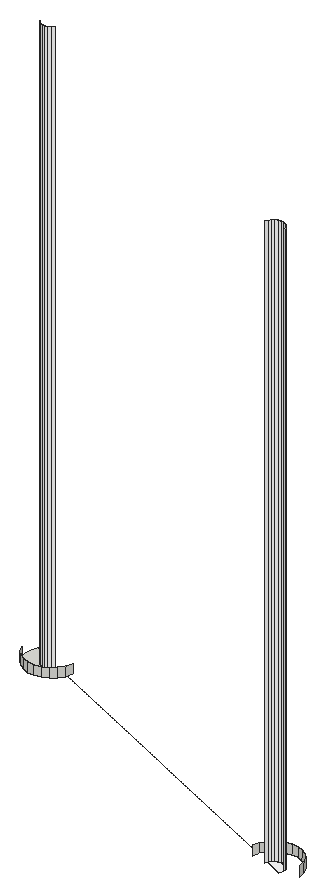
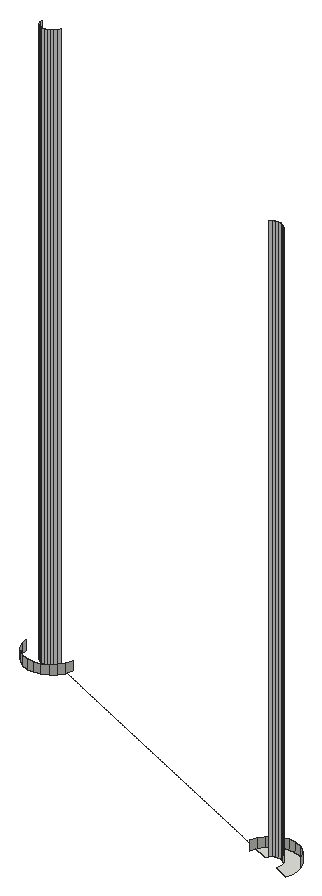
# SketchUp Ruby script. Lengths in inches.
U = 1.inch
M = Sketchup.active_model
def pt(a) = Geom::Point3d.new(a.map { |v| v * U })
def face(e, loops, mat)
  f = e.add_face(loops[0].map { |a| pt(a) })
  loops[1..].each { |l| e.add_face(l.map { |a| pt(a) }).erase! }
  f.material = f.back_material = mat if mat
  f
end
# faces: each face lists its corners as indices into pts; further lists are holes
def faces(e, pts, list, mat = nil) = list.each { |f| face(e, (f[0].is_a?(Array) ? f : [f]).map { |l| l.map { |i| pts[i] } }, mat) }
# xy, xz, yz: faces in a plane at the given z, y or x. An outline is a flat list of corners, or four numbers for a rectangle; further outlines are holes
def ring(l) = l.size == 4 ? [[l[0], l[1]], [l[2], l[1]], [l[2], l[3]], [l[0], l[3]]] : l.each_slice(2).to_a
def flat(e, list, mat, &to3) = list.each { |f| face(e, (f[0].is_a?(Array) ? f : [f]).map { |l| ring(l).map { |u, v| to3.(u, v) } }, mat) }
def xy(e, z, list, mat = nil) = flat(e, list, mat) { |x, y| [x, y, z] }
def xz(e, y, list, mat = nil) = flat(e, list, mat) { |x, z| [x, y, z] }
def yz(e, x, list, mat = nil) = flat(e, list, mat) { |y, z| [x, y, z] }
def lines(e, pts, list) = list.each { |a, b| e.add_line(pt(pts[a]), pt(pts[b])) }
# prism: a flat outline (further loops are holes) pulled along v
def prism(e, loops, v, mat = nil)
  f = face(e, loops, mat); d = Geom::Vector3d.new(v.map { |x| x * U })
  f.pushpull(f.normal.samedirection?(d) ? d.length : -d.length)
end
def box(e, o, s, mat = nil) = prism(e, [[o, [o[0] + s[0], o[1], o[2]], [o[0] + s[0], o[1] + s[1], o[2]], [o[0], o[1] + s[1], o[2]]]], [0, 0, s[2]], mat)
def at(x, y, z, deg = 0) = Geom::Transformation.translation(pt([x, y, z])) * Geom::Transformation.rotation(ORIGIN, Z_AXIS, deg.degrees)
def axes(o, x, y, z) = Geom::Transformation.new([*x, 0, *y, 0, *z, 0, *pt(o).to_a, 1])
def part(name) = M.definitions.add(name)
# library, detail: a bought-in or finely detailed component or shape, given as its bounding box
def library(name, o, s) = part(name).tap { |d| box(d.entities, o, s) }
def detail(e, o, s) = box(e.add_group.entities, o, s)
def put(e, d, t, mat = nil) = e.add_instance(d, t).tap { |i| i.material = mat if mat }
def group(e, t, mat = nil) = e.add_group.tap { |g| g.transformation = t; g.material = mat if mat }.entities
root = M.entities
M.materials.add("[Color_000]").color = [255, 255, 255]
xy(root,321.27,[[916.82,1057.59,916.41,1057.62,916.02,1057.75,915.68,1057.97,915.4,1058.28,915.22,1058.65,915.14,1059.05,915.16,1059.46,915.27,1059.79,916.13,1059.41,916.09,1059.28,916.08,1059.12,916.11,1058.96,916.1875,1058.81,916.3,1058.6875,916.43,1058.6,916.59,1058.54,916.75,1058.53,916.91,1058.57,917.0625,1058.64,917.18,1058.75,917.27,1058.89,917.28,1058.91,918.15,1058.54,918.125,1058.47,917.9,1058.13,917.59,1057.86,917.22,1057.67]])
xy(root,321.27,[[938.52,1049.66,937.37,1050.17,937.375,1050.19,937.47,1050.33,937.59,1050.4375,937.74,1050.51,937.9,1050.54,938.0625,1050.53,938.22,1050.48,938.35,1050.39,938.46,1050.27,938.54,1050.12,938.57,1049.96,938.56,1049.8]],"[Color_000]")
p = [[937.375,1050.19,321.27],[937.37,1050.17,321.27],[937.32,1050.03,321.27],[937.32,1050.03,357.27],[937.375,1050.19,357.27],[938.57,1049.96,321.27],
  [938.54,1050.12,321.27],[938.54,1050.12,357.27],[938.57,1049.96,357.27],[939.51,1050.03,321.27],[939.43,1050.43,321.27],[939.43,1050.43,321.86],
  [939.51,1050.03,321.86],[938.46,1050.27,321.27],[938.46,1050.27,357.27],[936.52,1050.6,321.27],[936.5,1050.54,321.27],[936.4,1050.21,321.27],
  [936.4,1050.21,321.86],[936.52,1050.6,321.86],[937.47,1050.33,321.27],[937.47,1050.33,357.27],[937.59,1050.4375,321.27],[937.59,1050.4375,357.27],
  [938.35,1050.39,321.27],[938.35,1050.39,357.27],[937.74,1050.51,321.27],[937.74,1050.51,357.27],[938.22,1050.48,321.27],[938.22,1050.48,357.27],
  [939.25,1050.8,321.27],[939.25,1050.8,321.86],[937.9,1050.54,321.27],[937.9,1050.54,357.27],[938.0625,1050.53,321.27],[938.0625,1050.53,357.27],
  [936.75,1050.95,321.27],[936.75,1050.95,321.86],[938.97,1051.11,321.27],[938.97,1051.11,321.86],[937.06,1051.22,321.27],[937.06,1051.22,321.86],
  [938.63,1051.33,321.27],[938.63,1051.33,321.86],[937.43,1051.4,321.27],[937.43,1051.4,321.86],[938.24,1051.46,321.27],[938.24,1051.46,321.86],
  [937.83,1051.49,321.27],[937.83,1051.49,321.86],[916.02,1057.75,321.27],[916.41,1057.62,321.27],[916.41,1057.62,321.86],[916.02,1057.75,321.86],
  [916.82,1057.59,321.27],[916.82,1057.59,321.86],[917.22,1057.67,321.27],[917.22,1057.67,321.86],[915.68,1057.97,321.27],[915.68,1057.97,321.86],
  [917.59,1057.86,321.27],[917.59,1057.86,321.86],[917.9,1058.13,321.27],[917.9,1058.13,321.86],[915.4,1058.28,321.27],[915.4,1058.28,321.86],
  [918.125,1058.47,321.27],[918.125,1058.47,321.86],[915.22,1058.65,321.27],[915.22,1058.65,321.86],[916.43,1058.6,321.27],[916.59,1058.54,321.27],
  [916.59,1058.54,357.27],[916.43,1058.6,357.27],[916.75,1058.53,321.27],[916.75,1058.53,357.27],[916.91,1058.57,321.27],[916.91,1058.57,357.27],
  [918.15,1058.54,321.27],[918.25,1058.86,321.27],[918.25,1058.86,321.86],[916.3,1058.6875,321.27],[916.3,1058.6875,357.27],[917.0625,1058.64,321.27],
  [917.0625,1058.64,357.27],[917.18,1058.75,321.27],[917.18,1058.75,357.27],[916.1875,1058.81,321.27],[916.1875,1058.81,357.27]]
faces(root,p,[[0,1,2,3,4],[5,6,7,8],[6,13,14,7],[20,0,4,21],[22,20,21,23],[13,24,25,14],[26,22,23,27],[24,28,29,25],
  [32,26,27,33],[34,32,33,35],[28,34,35,29],[70,71,72,73],[71,74,75,72],[74,76,77,75],[81,70,73,82],[76,83,84,77],
  [83,85,86,84],[87,81,82,88]],"[Color_000]")
faces(root,p,[[9,10,11,12],[15,16,17,18,19],[10,30,31,11],[36,15,19,37],[30,38,39,31],[40,36,37,41],[38,42,43,39],[44,40,41,45],
  [42,46,47,43],[48,44,45,49],[46,48,49,47],[50,51,52,53],[51,54,55,52],[54,56,57,55],[58,50,53,59],[56,60,61,57],
  [60,62,63,61],[64,58,59,65],[62,66,67,63],[68,64,65,69],[66,78,79,80,67]])
lines(root,p,[[16,78]])
